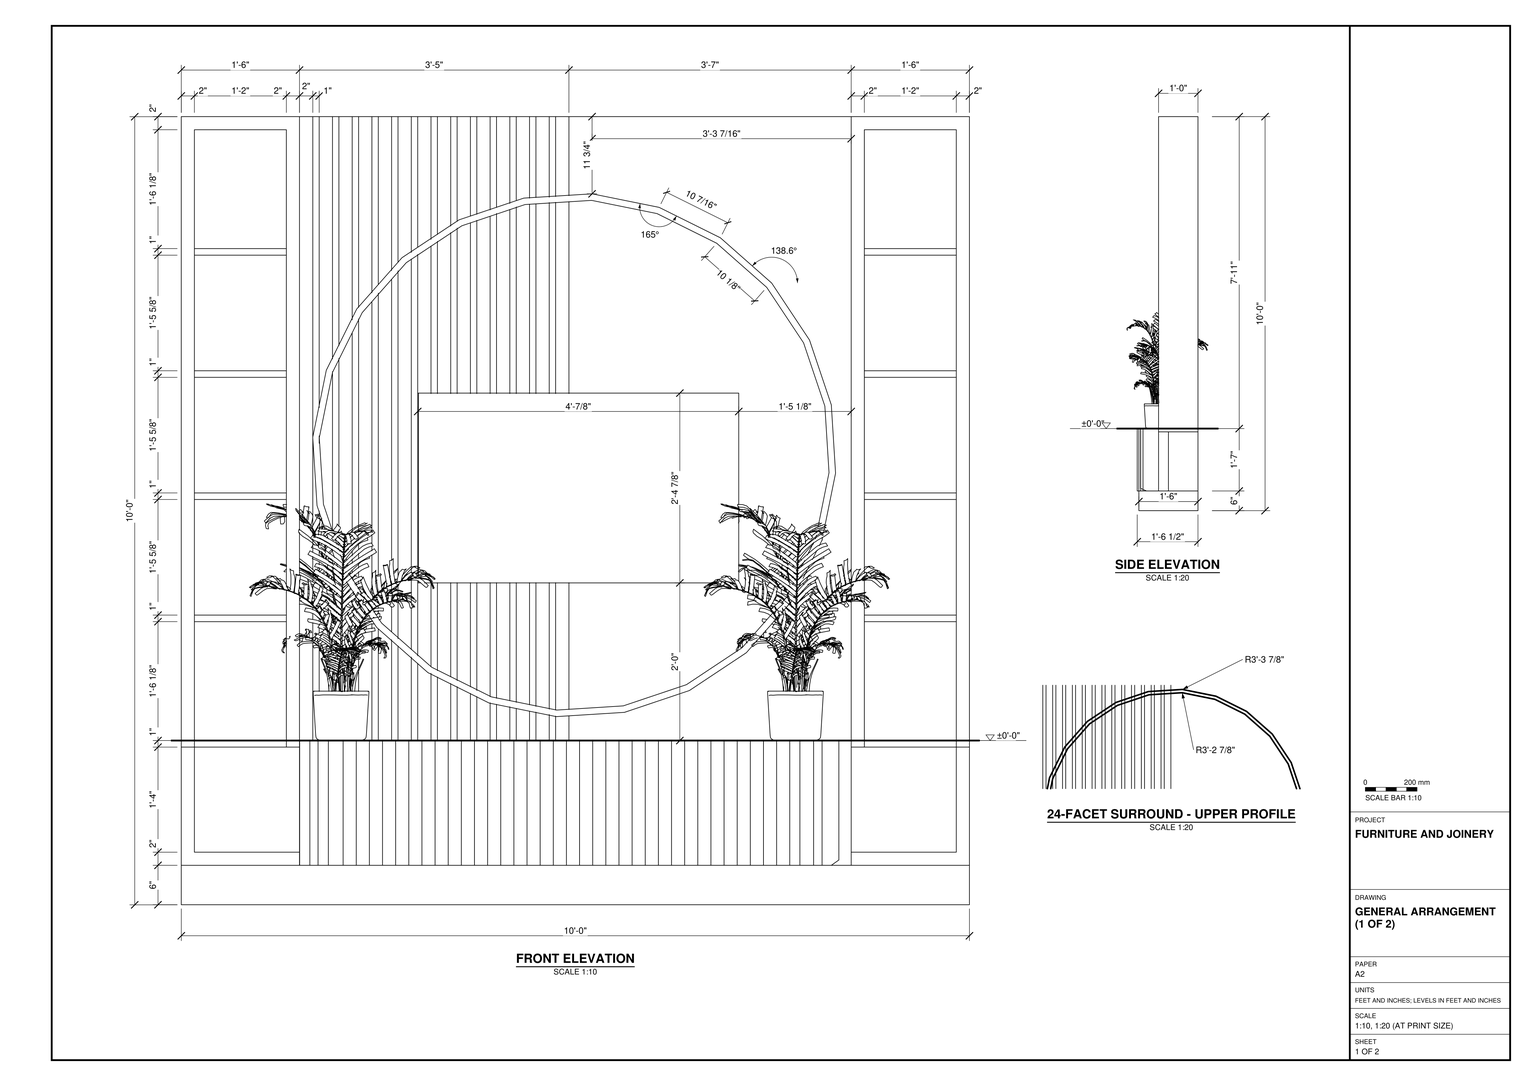
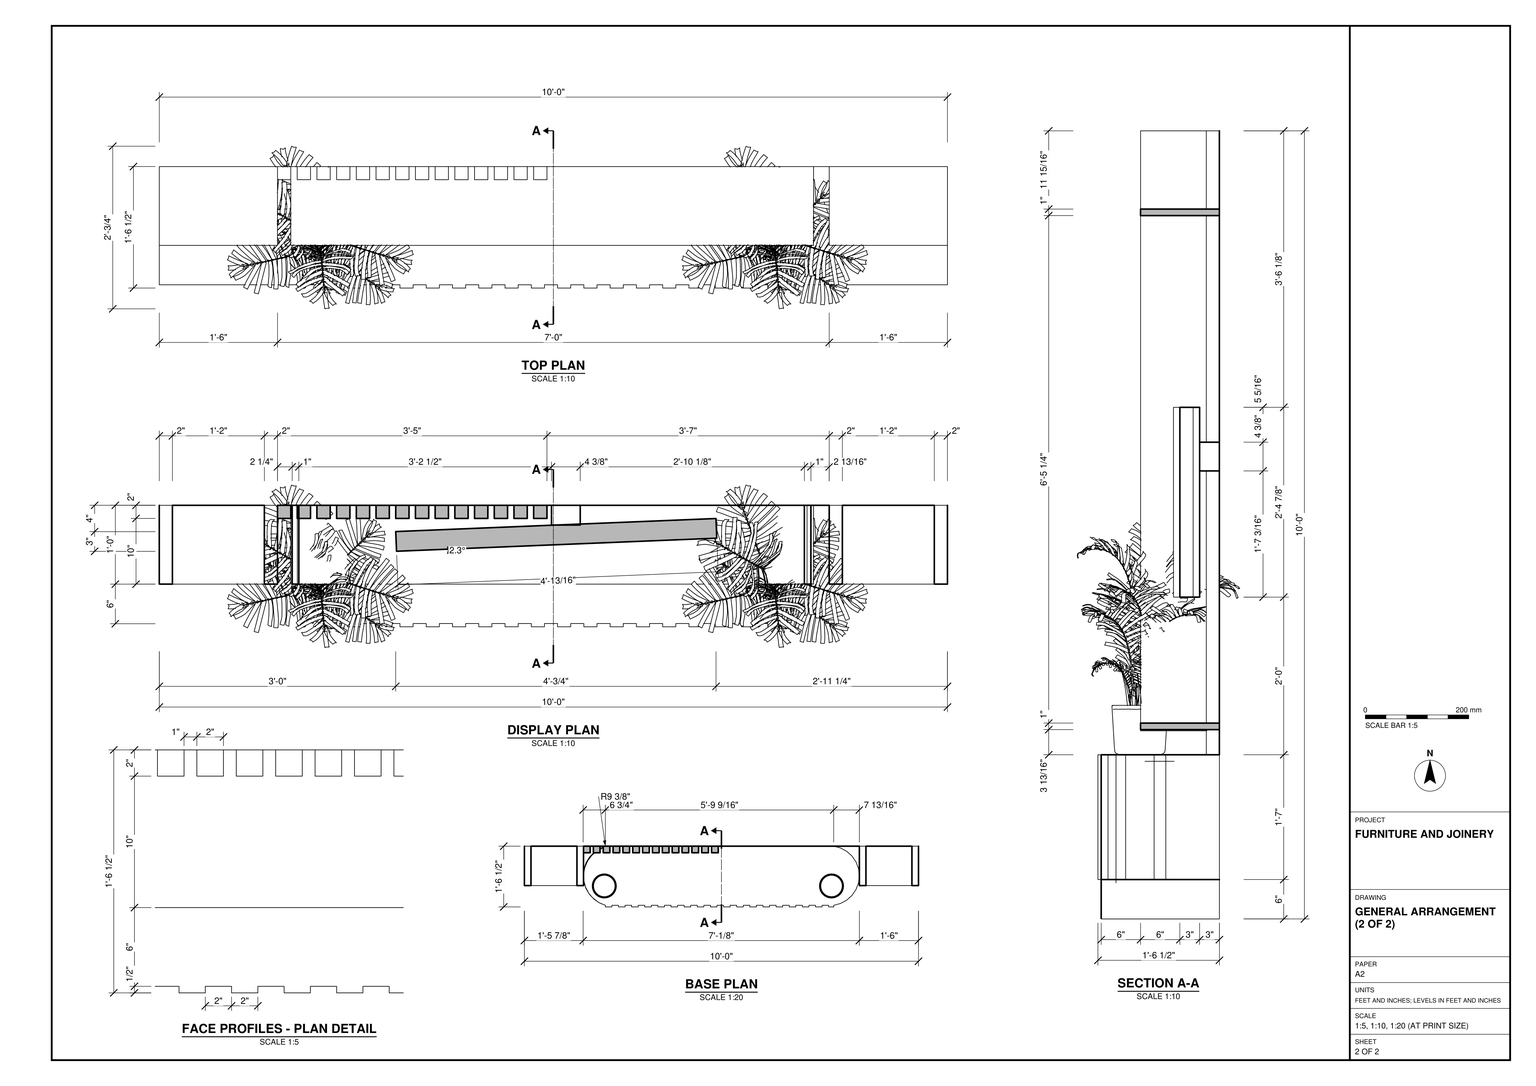
Build the display wall in SketchUp from task_files/diagram_01.pdf. Work in feet and inches. The complete assembly, including the plants, is 10'-0" wide, 2'-3/4" deep and 10'-0" high. Use the console top as the ±0'-0" reference shown in the elevations.

Frame the 7'-0" central bay with open shelving towers. Match their side thicknesses, shelf thicknesses and shelf elevations to the front view. Build the low plinth and the projecting console, following the rounded ends in the base plan and the stepped front edge in the face-profile detail. Above the console, model vertical slats on the left side of the bay and a plain backing on the right. Set the narrow, 24-sided surround across both surfaces. Position the rectangular display inside the surround, using the section for its height above the console and the display plan for its slight angle to the backing.

Place a potted plant on the console at each side of the display. Decor and loose items, including the plants, may be any suitable library components. Keep the joinery pieces, surround and display in separate groups or components, and use components for repeated parts. Save one SketchUp model as output_files/display_wall_with_shelving_and_a_faceted_surround.skp.

# SketchUp Ruby script. Lengths in inches.
U = 1.inch
M = Sketchup.active_model
def pt(a) = Geom::Point3d.new(a.map { |v| v * U })
def face(e, loops, mat)
  f = e.add_face(loops[0].map { |a| pt(a) })
  loops[1..].each { |l| e.add_face(l.map { |a| pt(a) }).erase! }
  f.material = f.back_material = mat if mat
  f
end
# faces: each face lists its corners as indices into pts; further lists are holes
def faces(e, pts, list, mat = nil) = list.each { |f| face(e, (f[0].is_a?(Array) ? f : [f]).map { |l| l.map { |i| pts[i] } }, mat) }
# xy, xz, yz: faces in a plane at the given z, y or x. An outline is a flat list of corners, or four numbers for a rectangle; further outlines are holes
def ring(l) = l.size == 4 ? [[l[0], l[1]], [l[2], l[1]], [l[2], l[3]], [l[0], l[3]]] : l.each_slice(2).to_a
def flat(e, list, mat, &to3) = list.each { |f| face(e, (f[0].is_a?(Array) ? f : [f]).map { |l| ring(l).map { |u, v| to3.(u, v) } }, mat) }
def xy(e, z, list, mat = nil) = flat(e, list, mat) { |x, y| [x, y, z] }
def xz(e, y, list, mat = nil) = flat(e, list, mat) { |x, z| [x, y, z] }
def yz(e, x, list, mat = nil) = flat(e, list, mat) { |y, z| [x, y, z] }
def lines(e, pts, list) = list.each { |a, b| e.add_line(pt(pts[a]), pt(pts[b])) }
# prism: a flat outline (further loops are holes) pulled along v
def prism(e, loops, v, mat = nil)
  f = face(e, loops, mat); d = Geom::Vector3d.new(v.map { |x| x * U })
  f.pushpull(f.normal.samedirection?(d) ? d.length : -d.length)
end
def box(e, o, s, mat = nil) = prism(e, [[o, [o[0] + s[0], o[1], o[2]], [o[0] + s[0], o[1] + s[1], o[2]], [o[0], o[1] + s[1], o[2]]]], [0, 0, s[2]], mat)
def at(x, y, z, deg = 0) = Geom::Transformation.translation(pt([x, y, z])) * Geom::Transformation.rotation(ORIGIN, Z_AXIS, deg.degrees)
def axes(o, x, y, z) = Geom::Transformation.new([*x, 0, *y, 0, *z, 0, *pt(o).to_a, 1])
def part(name) = M.definitions.add(name)
# library, detail: a bought-in or finely detailed component or shape, given as its bounding box
def library(name, o, s) = part(name).tap { |d| box(d.entities, o, s) }
def detail(e, o, s) = box(e.add_group.entities, o, s)
def put(e, d, t, mat = nil) = e.add_instance(d, t).tap { |i| i.material = mat if mat }
def group(e, t, mat = nil) = e.add_group.tap { |g| g.transformation = t; g.material = mat if mat }.entities
root = M.entities
M.materials.add("[0054_LightYellow]").color = [255, 255, 224]
M.materials.add("[0137_Black]").color = [0, 0, 0]
M.materials.add("[Carrera Marble]").color = [207, 207, 207]
M.materials.add("[Wood Floor Parquet]").color = [145, 89, 39]
M.materials.add("[Wood Veneer 01]").color = [120, 70, 37]
c1 = part("Group\#5")
box(c1.entities,[0,0,0],[2.03,2,95])
c2 = part("Display wall panel")
put(c2.entities,c1,at(15,0,0),"[Wood Veneer 01]")
put(c2.entities,c1,at(21,0,0),"[Wood Veneer 01]")
put(c2.entities,c1,at(24,0,0),"[Wood Veneer 01]")
put(c2.entities,c1,at(27,0,0),"[Wood Veneer 01]")
g1 = group(c2.entities,at(12,0,0),"[Wood Veneer 01]")
box(g1,[0,0,0],[2.03,2,95])
put(c2.entities,c1,at(39,0,0),"[Wood Veneer 01]")
g2 = group(c2.entities,at(6,0,0),"[Wood Veneer 01]")
box(g2,[0,0,0],[2.03,2,95])
put(c2.entities,c1,at(36,0,0),"[Wood Veneer 01]")
put(c2.entities,c1,at(9,0,0),"[Wood Veneer 01]")
put(c2.entities,c1,at(30,0,0),"[Wood Veneer 01]")
put(c2.entities,c1,at(33,0,0),"[Wood Veneer 01]")
put(c2.entities,c1,at(18,0,0),"[Wood Veneer 01]")
put(c2.entities,c1,at(0,0,0),"[Wood Veneer 01]")
g3 = group(c2.entities,at(3,0,0),"[Wood Veneer 01]")
box(g3,[0,0,0],[2.03,2,95])
c3 = library("SKT_Nearly Natural 5' Kentia Palm Silk Tree",[-23.18,-17.61,0],[47.48,43.95,59.125])
xy(root,96.46,[[59.72,15.49,64.09,18.49]],"[Carrera Marble]")
xy(root,100.84,[[59.72,15.49,64.09,18.49]],"[Carrera Marble]")
xz(root,6.49,[[[57.09,56.89,67.48,57.54,77.36,60.86,86.03,66.62,92.92,74.43,97.56,83.75,99.62,93.96,98.97,104.36,95.65,114.23,89.89,122.9,82.08,129.79,72.75,134.43,62.55,136.49,52.15,135.84,42.28,132.52,33.6,126.76,26.71,118.95,22.08,109.625,20.02,99.42,20.67,89.02,23.99,79.15,29.75,70.48,37.56,63.59,46.88,58.95],[57.16,57.89,47.21,59.9,38.11,64.42,30.5,71.13,24.88,79.59,21.65,89.22,21.02,99.35,23.03,109.3,27.54,118.39,34.26,126.01,42.72,131.625,52.34,134.86,62.48,135.49,72.43,133.48,81.52,128.96,89.14,122.25,94.75,113.79,97.99,104.16,98.62,94.03,96.61,84.08,92.09,74.99,85.375,67.37,76.92,61.76,67.29,58.52]]],"[Wood Veneer 01]")
xz(root,18.49,[[[57.09,56.89,46.88,58.95,37.56,63.59,29.75,70.48,23.99,79.15,20.67,89.02,20.02,99.42,22.08,109.625,26.71,118.95,33.6,126.76,42.28,132.52,52.15,135.84,62.55,136.49,72.75,134.43,82.08,129.79,89.89,122.9,95.65,114.23,98.97,104.36,99.62,93.96,97.56,83.75,92.92,74.43,86.03,66.62,77.36,60.86,67.48,57.54],[57.16,57.89,67.29,58.52,76.92,61.76,85.375,67.37,92.09,74.99,96.61,84.08,98.62,94.03,97.99,104.16,94.75,113.79,89.14,122.25,81.52,128.96,72.43,133.48,62.48,135.49,52.34,134.86,42.72,131.625,34.26,126.01,27.54,118.39,23.03,109.3,21.02,99.35,21.65,89.22,24.88,79.59,30.5,71.13,38.11,64.42,47.21,59.9]]])
xz(root,18.49,[[[57.16,57.89,67.29,58.52,76.92,61.76,85.375,67.37,92.09,74.99,96.61,84.08,98.62,94.03,97.99,104.16,94.75,113.79,89.14,122.25,81.52,128.96,72.43,133.48,62.48,135.49,52.34,134.86,42.72,131.625,34.26,126.01,27.54,118.39,23.03,109.3,21.02,99.35,21.65,89.22,24.88,79.59,30.5,71.13,38.11,64.42,47.21,59.9],[59.72,96.46,64.09,100.84]]],"[Carrera Marble]")
xz(root,18.5,[[59.03,53.25,102,148.25]],"[Carrera Marble]")
yz(root,59.72,[[15.49,96.46,18.49,100.84]],"[Carrera Marble]")
yz(root,64.09,[[15.49,96.46,18.49,100.84]],"[Carrera Marble]")
p = [[46.88,18.49,58.95],[57.09,18.49,56.89],[57.09,6.49,56.89],[46.88,6.49,58.95],[67.48,18.49,57.54],[67.48,6.49,57.54],
  [77.36,18.49,60.86],[77.36,6.49,60.86],[57.16,18.49,57.89],[47.21,18.49,59.9],[47.21,6.49,59.9],[57.16,6.49,57.89],
  [67.29,18.49,58.52],[67.29,6.49,58.52],[76.92,18.49,61.76],[76.92,6.49,61.76],[37.56,18.49,63.59],[37.56,6.49,63.59],
  [38.11,18.49,64.42],[38.11,6.49,64.42],[86.03,18.49,66.62],[86.03,6.49,66.62],[85.375,18.49,67.37],[85.375,6.49,67.37],
  [29.75,18.49,70.48],[29.75,6.49,70.48],[30.5,18.49,71.13],[30.5,6.49,71.13],[92.92,18.49,74.43],[92.92,6.49,74.43],
  [92.09,18.49,74.99],[92.09,6.49,74.99],[23.99,18.49,79.15],[23.99,6.49,79.15],[24.88,18.49,79.59],[24.88,6.49,79.59],
  [97.56,18.49,83.75],[97.56,6.49,83.75],[96.61,18.49,84.08],[96.61,6.49,84.08],[20.67,18.49,89.02],[20.67,6.49,89.02],
  [21.65,18.49,89.22],[21.65,6.49,89.22],[99.62,18.49,93.96],[99.62,6.49,93.96],[98.62,18.49,94.03],[98.62,6.49,94.03],
  [20.02,18.49,99.42],[20.02,6.49,99.42],[21.02,18.49,99.35],[21.02,6.49,99.35],[97.99,18.49,104.16],[97.99,6.49,104.16],
  [98.97,18.49,104.36],[98.97,6.49,104.36],[23.03,18.49,109.3],[23.03,6.49,109.3],[22.08,18.49,109.625],[22.08,6.49,109.625],
  [94.75,18.49,113.79],[94.75,6.49,113.79],[95.65,18.49,114.23],[95.65,6.49,114.23],[27.54,18.49,118.39],[27.54,6.49,118.39],
  [26.71,18.49,118.95],[26.71,6.49,118.95],[89.14,18.49,122.25],[89.14,6.49,122.25],[89.89,18.49,122.9],[89.89,6.49,122.9],
  [34.26,18.49,126.01],[34.26,6.49,126.01],[33.6,18.49,126.76],[33.6,6.49,126.76],[81.52,18.49,128.96],[81.52,6.49,128.96],
  [82.08,18.49,129.79],[82.08,6.49,129.79],[42.72,18.49,131.625],[42.72,6.49,131.625],[42.28,18.49,132.52],[42.28,6.49,132.52],
  [72.43,18.49,133.48],[72.43,6.49,133.48],[72.75,18.49,134.43],[72.75,6.49,134.43],[52.34,18.49,134.86],[52.34,6.49,134.86],
  [52.15,18.49,135.84],[52.15,6.49,135.84],[62.48,18.49,135.49],[62.48,6.49,135.49],[62.55,18.49,136.49],[62.55,6.49,136.49],
  [59.82,18.49,53.27],[60.18,18.5,53.27],[94.1875,0.5,53.25],[96.28,1.06,53.25],[98.17,2.09,53.25],[99.77,3.54,53.25],
  [100.99,5.33,53.25],[101.74,7.35,53.25],[102,9.5,53.25],[101.74,11.65,53.25],[100.99,13.67,53.25],[99.77,15.46,53.25],
  [98.17,16.91,53.25],[96.28,17.94,53.25],[94.1875,18.5,53.25],[24.64,0.5,53.25],[22.79,1.27,53.25],[21.14,2.41,53.25],
  [19.77,3.875,53.25],[18.74,5.6,53.25],[18.11,7.5,53.25],[17.89,9.5,53.25],[18.11,11.5,53.25],[18.74,13.4,53.25],
  [19.77,15.125,53.25],[21.14,16.59,53.25],[22.79,17.73,53.25],[24.64,18.5,53.25],[97.5625,1.76,34.25],[97.5625,1.76,53.25],
  [100.12,1.01,53.25],[100.12,1.01,35.06],[96.28,1.06,34.25]]
faces(root,p,[[0,1,2,3],[1,4,5,2],[4,6,7,5],[8,9,10,11],[12,8,11,13],[14,12,13,15],[16,0,3,17],[9,18,19,10],
  [6,20,21,7],[22,14,15,23],[24,16,17,25],[18,26,27,19],[20,28,29,21],[30,22,23,31],[32,24,25,33],[26,34,35,27],
  [28,36,37,29],[38,30,31,39],[40,32,33,41],[34,42,43,35],[36,44,45,37],[46,38,39,47],[48,40,41,49],[42,50,51,43],
  [52,46,47,53],[44,54,55,45],[50,56,57,51],[58,48,49,59],[60,52,53,61],[54,62,63,55],[56,64,65,57],[66,58,59,67],
  [68,60,61,69],[62,70,71,63],[64,72,73,65],[74,66,67,75],[76,68,69,77],[70,78,79,71],[72,80,81,73],[82,74,75,83],
  [84,76,77,85],[78,86,87,79],[80,88,89,81],[90,82,83,91],[92,84,85,93],[86,94,95,87],[88,92,93,89],[94,90,91,95]],"[Wood Veneer 01]")
lines(root,p,[[96,97],[98,99],[100,101],[101,102],[102,103],[103,104],[104,105],[105,106],[106,107],[107,108],[108,109],[109,110],
  [111,112],[112,113],[113,114],[114,115],[115,116],[116,117],[117,118],[118,119],[119,120],[120,121],[121,122],[122,123],
  [124,125],[126,127],[128,99],[99,125],[125,100]])
put(root,c2,at(18,16.5,53.25))
put(root,c3,axes([93.49,6.31,53.25],[0.65,0,0],[0,0.65,0],[0,0,0.65]))
put(root,c3,axes([24.3,6.31,53.25],[0.65,0,0],[0,0.65,0],[0,0,0.65]))
put(root,c1,at(21,16.5,53.25),"[Wood Veneer 01]")
put(root,c1,at(24,16.5,53.25),"[Wood Veneer 01]")
put(root,c1,at(30,16.5,53.25),"[Wood Veneer 01]")
put(root,c1,at(36,16.5,53.25),"[Wood Veneer 01]")
put(root,c1,at(42,16.5,53.25),"[Wood Veneer 01]")
put(root,c1,at(48,16.5,53.25),"[Wood Veneer 01]")
put(root,c1,at(54,16.5,53.25),"[Wood Veneer 01]")
put(root,c1,at(51,16.5,53.25),"[Wood Veneer 01]")
g4 = group(root,at(0,18.5,28.25),"[Wood Floor Parquet]")
xy(g4,6,[[0,-18,18,0],[24.64,-18,22.84,-17.26,22.4,-16.96,20.82,-15.75,19.88,-14.77,19.58,-14.28,18.65,-12.55,18.11,-10.53,18.03,-8.4375,18.42,-6.38,19.27,-4.47,20.53,-2.8,22.13,-1.46,24,-0.51,26.03,0,94.1875,0,96.28,-0.56,98.17,-1.59,99.77,-3.04,100.99,-4.83,101.74,-6.85,102,-9,101.74,-11.15,100.99,-13.17,99.77,-14.96,98.97,-15.68,98.17,-16.41,97.5625,-16.74,96.28,-17.44,94.1875,-18],[102,-18,120,0],[22.4,-16.96,21.23,-16.17,20.82,-15.75]])
xy(g4,6,[[24.64,-18.5,26.64,-18],[28.64,-18.5,30.64,-18],[32.64,-18.5,34.64,-18],[36.64,-18.5,38.64,-18],[40.64,-18.5,42.64,-18],
  [44.64,-18.5,46.64,-18],[48.64,-18.5,50.64,-18],[52.64,-18.5,54.64,-18],[56.64,-18.5,58.64,-18],[60.64,-18.5,62.64,-18],
  [64.64,-18.5,66.64,-18],[68.64,-18.5,70.64,-18],[72.64,-18.5,74.64,-18],[76.64,-18.5,78.64,-18],[80.64,-18.5,82.64,-18],
  [84.64,-18.5,86.64,-18],[88.64,-18.5,90.64,-18],[92.64,-18.5,94.1875,-18]],"[0054_LightYellow]")
xy(g4,24,[[0,-12,2,0],[102,-12,104,0],[104,-12,118,0],[118,-12,120,0]])
xy(g4,24,[[2,-12,16,0],[16,-12,18,0]],"[Wood Floor Parquet]")
xy(g4,25,[[22.77,-17.21,22.4,-16.96,22.71,-17.19],[21.08,-16.01,20.82,-15.75,21.02,-15.97],[19.67,-14.43,19.58,-14.28,19.64,-14.39],[18,-9.94,18,-8.16,17.92,-9.36]])
xy(g4,25,[[24.64,-18.5,26.64,-18.5,26.64,-18,28.64,-18,28.64,-18.5,30.64,-18.5,30.64,-18,32.64,-18,32.64,-18.5,34.64,-18.5,34.64,-18,36.64,-18,36.64,-18.5,38.64,-18.5,38.64,-18,40.64,-18,40.64,-18.5,42.64,-18.5,42.64,-18,44.64,-18,44.64,-18.5,46.64,-18.5,46.64,-18,48.64,-18,48.64,-18.5,50.64,-18.5,50.64,-18,52.64,-18,52.64,-18.5,54.64,-18.5,54.64,-18,56.64,-18,56.64,-18.5,58.64,-18.5,58.64,-18,60.64,-18,60.64,-18.5,62.64,-18.5,62.64,-18,64.64,-18,64.64,-18.5,66.64,-18.5,66.64,-18,68.64,-18,68.64,-18.5,70.64,-18.5,70.64,-18,72.64,-18,72.64,-18.5,74.64,-18.5,74.64,-18,76.64,-18,76.64,-18.5,78.64,-18.5,78.64,-18,80.64,-18,80.64,-18.5,82.64,-18.5,82.64,-18,84.64,-18,84.64,-18.5,86.64,-18.5,86.64,-18,88.64,-18,88.64,-18.5,90.64,-18.5,90.64,-18,92.64,-18,92.64,-18.5,94.1875,-18.5,94.1875,-18,96.28,-17.44,97.5625,-16.74,98.17,-16.41,99.77,-14.96,100.99,-13.17,101.74,-11.15,102,-9,101.74,-6.85,100.99,-4.83,99.77,-3.04,98.17,-1.59,96.28,-0.56,94.1875,0,26.03,0,24,-0.51,22.13,-1.46,20.53,-2.8,19.27,-4.47,18.42,-6.38,18.03,-8.4375,18.11,-10.53,18.65,-12.55,19.58,-14.28,19.67,-14.43,20.82,-15.75,22.4,-16.96,22.77,-17.21,24.64,-18],[24.64,-18,22.77,-17.21,22.84,-17.26],[22.4,-16.96,20.82,-15.75,21.08,-16.01],[22.4,-16.96,21.08,-16.01,21.23,-16.17],[20.82,-15.75,19.67,-14.43,19.88,-14.77],
  [2,-12,16,0],[104,-12,118,0]],"[Wood Veneer 01]")
xy(g4,43.1,[[2,-12,16,0]],"[Wood Floor Parquet]")
xy(g4,43.1,[[104,-12,118,0]],"[Wood Veneer 01]")
xy(g4,44.1,[[2,-12,16,0],[104,-12,118,0]],"[Wood Veneer 01]")
xy(g4,61.7,[[2,-12,16,0]])
xy(g4,61.7,[[104,-12,118,0]],"[Wood Veneer 01]")
xy(g4,62.7,[[2,-12,16,0],[104,-12,118,0]],"[Wood Veneer 01]")
xy(g4,80.3,[[2,-12,16,0]])
xy(g4,80.3,[[104,-12,118,0]],"[Wood Veneer 01]")
xy(g4,81.3,[[2,-12,16,0],[104,-12,118,0]],"[Wood Veneer 01]")
xy(g4,98.9,[[2,-12,16,0],[104,-12,118,0]])
xy(g4,99.9,[[2,-12,16,0],[104,-12,118,0]],"[Wood Veneer 01]")
xy(g4,118,[[2,-12,16,0],[104,-12,118,0]])
xy(g4,120,[[0,-12,18,0],[102,-12,120,0]],"[Wood Veneer 01]")
xz(g4,-18.5,[[24.64,6,26.64,25],[28.64,6,30.64,25],[32.64,6,34.64,25],[36.64,6,38.64,25],[40.64,6,42.64,25],
  [44.64,6,46.64,25],[48.64,6,50.64,25],[52.64,6,54.64,25],[56.64,6,58.64,25],[60.64,6,62.64,25],
  [64.64,6,66.64,25],[68.64,6,70.64,25],[72.64,6,74.64,25],[76.64,6,78.64,25],[80.64,6,82.64,25],
  [84.64,6,86.64,25],[88.64,6,90.64,25],[92.64,6,94.1875,25]],"[Wood Floor Parquet]")
xz(g4,-18,[[0,0,120,6]])
xz(g4,-18,[[26.64,6,28.64,25],[30.64,6,32.64,25],[34.64,6,36.64,25],[38.64,6,40.64,25],[42.64,6,44.64,25],
  [46.64,6,48.64,25],[50.64,6,52.64,25],[54.64,6,56.64,25],[58.64,6,60.64,25],[62.64,6,64.64,25],
  [66.64,6,68.64,25],[70.64,6,72.64,25],[74.64,6,76.64,25],[78.64,6,80.64,25],[82.64,6,84.64,25],
  [86.64,6,88.64,25],[90.64,6,92.64,25]],"[0054_LightYellow]")
xz(g4,-12,[[2,24,16,25]],"[Wood Floor Parquet]")
xz(g4,-12,[[0,24,2,24,2,118,16,118,16,24,18,24,18,120,0,120],[102,24,104,24,104,118,118,118,118,24,120,24,120,120,102,120],[104,24,118,25],[2,43.1,16,44.1],[104,43.1,118,44.1],
  [2,61.7,16,62.7],[104,61.7,118,62.7],[2,80.3,16,81.3],[104,80.3,118,81.3],[2,98.9,16,99.9],
  [104,98.9,118,99.9]],"[Wood Veneer 01]")
xz(g4,0,[[0,6,18,6,18,8,2,8,2,24,0,24],[18,6,26.03,6,26.03,25,94.1875,25,94.1875,6,102,6,102,120,18,120],[102,6,120,6,120,24,118,24,118,8,102,8],[102,8,118,24]])
xz(g4,0,[[2,8,18,24]],"[Wood Floor Parquet]")
xz(g4,0,[[2,25,16,43.1],[104,25,118,43.1],[2,44.1,16,61.7],[104,44.1,118,61.7],[2,62.7,16,80.3],
  [104,62.7,118,80.3],[2,81.3,16,98.9],[104,81.3,118,98.9],[2,99.9,16,118],[104,99.9,118,118]],"[Wood Veneer 01]")
yz(g4,0,[[-18,0,0,6],[-12,24,0,120]])
yz(g4,2,[[-12,25,0,43.1],[-12,44.1,0,61.7],[-12,62.7,0,80.3],[-12,81.3,0,98.9],[-12,99.9,0,118]],"[Wood Veneer 01]")
yz(g4,16,[[-12,25,0,43.1],[-12,44.1,0,61.7],[-12,62.7,0,80.3],[-12,81.3,0,98.9],[-12,99.9,0,118]],"[Wood Veneer 01]")
yz(g4,18,[[-12,6,-9.94,24],[-9.94,6,-8.16,24],[-8.16,6,0,24],[-12,24,-9.94,24,-9.94,25,-8.16,25,-8.16,24,0,24,0,120,-12,120]],"[Wood Floor Parquet]")
yz(g4,18,[[-9.94,24,-8.16,25]],"[Wood Veneer 01]")
yz(g4,24.64,[[-18.5,6,-18,25]],"[0054_LightYellow]")
yz(g4,26.64,[[-18.5,6,-18,25]],"[0054_LightYellow]")
yz(g4,28.64,[[-18.5,6,-18,25]],"[0054_LightYellow]")
yz(g4,30.64,[[-18.5,6,-18,25]],"[0054_LightYellow]")
yz(g4,32.64,[[-18.5,6,-18,25]],"[0054_LightYellow]")
yz(g4,34.64,[[-18.5,6,-18,25]],"[0054_LightYellow]")
yz(g4,36.64,[[-18.5,6,-18,25]],"[0054_LightYellow]")
yz(g4,38.64,[[-18.5,6,-18,25]],"[0054_LightYellow]")
yz(g4,40.64,[[-18.5,6,-18,25]],"[0054_LightYellow]")
yz(g4,42.64,[[-18.5,6,-18,25]],"[0054_LightYellow]")
yz(g4,44.64,[[-18.5,6,-18,25]],"[0054_LightYellow]")
yz(g4,46.64,[[-18.5,6,-18,25]],"[0054_LightYellow]")
yz(g4,48.64,[[-18.5,6,-18,25]],"[0054_LightYellow]")
yz(g4,50.64,[[-18.5,6,-18,25]],"[0054_LightYellow]")
yz(g4,52.64,[[-18.5,6,-18,25]],"[0054_LightYellow]")
yz(g4,54.64,[[-18.5,6,-18,25]],"[0054_LightYellow]")
yz(g4,56.64,[[-18.5,6,-18,25]],"[0054_LightYellow]")
yz(g4,58.64,[[-18.5,6,-18,25]],"[0054_LightYellow]")
yz(g4,60.64,[[-18.5,6,-18,25]],"[0054_LightYellow]")
yz(g4,62.64,[[-18.5,6,-18,25]],"[0054_LightYellow]")
yz(g4,64.64,[[-18.5,6,-18,25]],"[0054_LightYellow]")
yz(g4,66.64,[[-18.5,6,-18,25]],"[0054_LightYellow]")
yz(g4,68.64,[[-18.5,6,-18,25]],"[0054_LightYellow]")
yz(g4,70.64,[[-18.5,6,-18,25]],"[0054_LightYellow]")
yz(g4,72.64,[[-18.5,6,-18,25]],"[0054_LightYellow]")
yz(g4,74.64,[[-18.5,6,-18,25]],"[0054_LightYellow]")
yz(g4,76.64,[[-18.5,6,-18,25]],"[0054_LightYellow]")
yz(g4,78.64,[[-18.5,6,-18,25]],"[0054_LightYellow]")
yz(g4,80.64,[[-18.5,6,-18,25]],"[0054_LightYellow]")
yz(g4,82.64,[[-18.5,6,-18,25]],"[0054_LightYellow]")
yz(g4,84.64,[[-18.5,6,-18,25]],"[0054_LightYellow]")
yz(g4,86.64,[[-18.5,6,-18,25]],"[0054_LightYellow]")
yz(g4,88.64,[[-18.5,6,-18,25]],"[0054_LightYellow]")
yz(g4,90.64,[[-18.5,6,-18,25]],"[0054_LightYellow]")
yz(g4,92.64,[[-18.5,6,-18,25]],"[0054_LightYellow]")
yz(g4,94.1875,[[-18.5,6,-18,25]],"[0054_LightYellow]")
yz(g4,102,[[-12,6,-9,24],[-9,6,0,24]],"[Wood Floor Parquet]")
yz(g4,102,[[-12,24,0,120]],"[Wood Veneer 01]")
yz(g4,104,[[-12,99.9,0,118]])
yz(g4,104,[[-12,25,0,43.1],[-12,44.1,0,61.7],[-12,62.7,0,80.3],[-12,81.3,0,98.9]],"[Wood Veneer 01]")
yz(g4,118,[[-12,25,0,43.1],[-12,44.1,0,61.7],[-12,62.7,0,80.3],[-12,81.3,0,98.9],[-12,99.9,0,118]],"[Wood Veneer 01]")
yz(g4,120,[[-18,0,0,6],[-12,24,0,120]])
p = [[24.64,-18,25],[22.84,-17.26,25],[22.84,-17.26,6],[24.64,-18,6],[96.28,-17.44,25],[94.1875,-18,25],
  [94.1875,-18,6],[96.28,-17.44,6],[96.28,-17.44,6.4375],[97.5625,-16.74,6],[97.5625,-16.74,25],[22.77,-17.21,25],
  [22.4,-16.96,25],[22.4,-16.96,6],[20.82,-15.75,25],[20.82,-15.75,6],[21.23,-16.17,6],[21.23,-16.17,25],
  [98.17,-16.41,25],[98.17,-16.41,6],[99.77,-14.96,25],[98.97,-15.68,6],[99.77,-14.96,6],[21.08,-16.01,25],
  [19.88,-14.77,6],[19.88,-14.77,25],[100.99,-13.17,25],[100.99,-13.17,6],[19.58,-14.28,25],[19.58,-14.28,6],
  [19.67,-14.43,25],[18.65,-12.55,25],[18.65,-12.55,6],[101.74,-11.15,25],[101.74,-11.15,6],[18.11,-10.53,25],
  [18.11,-10.53,6],[102,-9,25],[102,-9,6],[102,-9,24],[18.03,-8.4375,25],[18.03,-8.4375,6],
  [101.74,-6.85,25],[101.74,-6.85,6],[18.42,-6.38,25],[18.42,-6.38,6],[100.99,-4.83,25],[100.99,-4.83,6],
  [19.27,-4.47,25],[19.27,-4.47,6],[99.77,-3.04,25],[99.77,-3.04,6],[20.53,-2.8,25],[20.53,-2.8,6],
  [98.17,-1.59,25],[98.17,-1.59,6],[22.13,-1.46,25],[22.13,-1.46,6],[96.28,-0.56,25],[96.28,-0.56,6],
  [24,-0.51,25],[24,-0.51,6],[94.1875,0,25],[94.1875,0,6],[26.03,0,25],[26.03,0,6],
  [120,0,0],[0,0,0],[18.05,-7.42,25],[18.58,-5.55,25],[19.49,-3.83,25],[20.73,-2.34,25],
  [22.26,-1.13,25],[24,-0.26,25],[18,-8.16,25],[20.82,-15.75,5.5],[100.12,-17.49,6.8125]]
faces(g4,p,[[0,1,2,3],[4,5,6,7,8],[11,12,13,2,1],[18,10,9,19],[20,18,19,21,22],[24,15,14,25],[26,20,22,27],[28,29,24,25,30],
  [28,31,32,29],[33,26,27,34],[31,35,36,32],[37,33,34,38,39],[35,40,41,36],[40,44,45,41],[44,48,49,45],[48,52,53,49],
  [52,56,57,53],[56,60,61,57],[60,64,65,61]],"[0054_LightYellow]")
faces(g4,p,[[7,9,10,4,8],[16,13,12,17],[23,14,15,16,17]],"[Wood Floor Parquet]")
faces(g4,p,[[13,12,14,15]])
faces(g4,p,[[42,37,39,38,43],[46,42,43,47],[50,46,47,51],[54,50,51,55],[58,54,55,59],[62,58,59,63]],"[Wood Veneer 01]")
lines(g4,p,[[66,67],[68,69],[69,70],[70,71],[71,72],[72,73],[74,68],[15,75],[76,21]])
g5 = group(root,at(59.72,15.49,96.46))
xz(g5,0,[[0,0,4.375,4.375]],"[Carrera Marble]")
g6 = group(root,at(36,11.5,77.25),"[0137_Black]")
prism(g6,[[[0,3,0],[48.75,4.99,0],[48.88,1.99,0],[0.12,0,0]]],[0,0,28.9])
